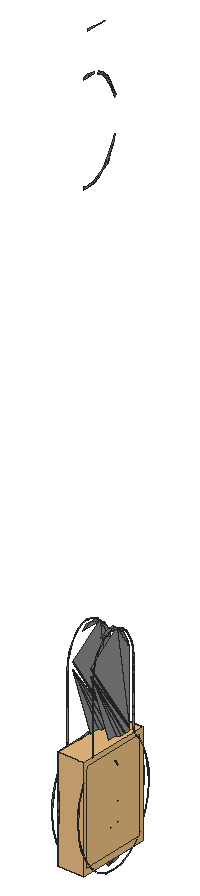
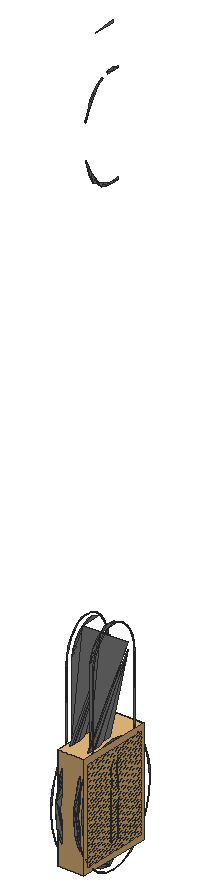
# SketchUp Ruby script. Lengths in inches.
U = 1.inch
M = Sketchup.active_model
def pt(a) = Geom::Point3d.new(a.map { |v| v * U })
def face(e, loops, mat)
  f = e.add_face(loops[0].map { |a| pt(a) })
  loops[1..].each { |l| e.add_face(l.map { |a| pt(a) }).erase! }
  f.material = f.back_material = mat if mat
  f
end
# faces: each face lists its corners as indices into pts; further lists are holes
def faces(e, pts, list, mat = nil) = list.each { |f| face(e, (f[0].is_a?(Array) ? f : [f]).map { |l| l.map { |i| pts[i] } }, mat) }
# xy, xz, yz: faces in a plane at the given z, y or x. An outline is a flat list of corners, or four numbers for a rectangle; further outlines are holes
def ring(l) = l.size == 4 ? [[l[0], l[1]], [l[2], l[1]], [l[2], l[3]], [l[0], l[3]]] : l.each_slice(2).to_a
def flat(e, list, mat, &to3) = list.each { |f| face(e, (f[0].is_a?(Array) ? f : [f]).map { |l| ring(l).map { |u, v| to3.(u, v) } }, mat) }
def xy(e, z, list, mat = nil) = flat(e, list, mat) { |x, y| [x, y, z] }
def xz(e, y, list, mat = nil) = flat(e, list, mat) { |x, z| [x, y, z] }
def yz(e, x, list, mat = nil) = flat(e, list, mat) { |y, z| [x, y, z] }
def lines(e, pts, list) = list.each { |a, b| e.add_line(pt(pts[a]), pt(pts[b])) }
# prism: a flat outline (further loops are holes) pulled along v
def prism(e, loops, v, mat = nil)
  f = face(e, loops, mat); d = Geom::Vector3d.new(v.map { |x| x * U })
  f.pushpull(f.normal.samedirection?(d) ? d.length : -d.length)
end
def box(e, o, s, mat = nil) = prism(e, [[o, [o[0] + s[0], o[1], o[2]], [o[0] + s[0], o[1] + s[1], o[2]], [o[0], o[1] + s[1], o[2]]]], [0, 0, s[2]], mat)
def at(x, y, z, deg = 0) = Geom::Transformation.translation(pt([x, y, z])) * Geom::Transformation.rotation(ORIGIN, Z_AXIS, deg.degrees)
def axes(o, x, y, z) = Geom::Transformation.new([*x, 0, *y, 0, *z, 0, *pt(o).to_a, 1])
def part(name) = M.definitions.add(name)
# library, detail: a bought-in or finely detailed component or shape, given as its bounding box
def library(name, o, s) = part(name).tap { |d| box(d.entities, o, s) }
def detail(e, o, s) = box(e.add_group.entities, o, s)
def put(e, d, t, mat = nil) = e.add_instance(d, t).tap { |i| i.material = mat if mat }
def group(e, t, mat = nil) = e.add_group.tap { |g| g.transformation = t; g.material = mat if mat }.entities
root = M.entities
M.materials.add("Material \#1").color = [140, 140, 140]
c1 = library("3DGeom~13_Defintion",[-84.91,-744.98,-830.03],[169.82,169.83,1000])
c2 = library("3DGeom~12_Defintion",[-95.68,-755.75,-830.03],[191.36,191.37,1000])
c3 = part("3DGeom~10_Defintion")
yz(c3.entities,-68.96,[[-797.08,-844.83,-797.08,-827.59,-922.41,-827.59],[-922.41,-844.83,-797.08,-844.83,-922.41,-827.59]],"Material \#1")
yz(c3.entities,68.97,[[-922.41,-844.83,-797.08,-827.59,-797.08,-844.83],[-922.41,-844.83,-922.41,-827.59,-797.08,-827.59],[-797.08,137.93,-922.41,155.17,-797.08,155.17],[-922.41,137.93,-922.41,155.17,-797.08,137.93]],"Material \#1")
p = [[-15.8,-989.55,-844.83],[-15.8,-989.55,-827.59],[0,-991.38,-827.59],[0,-991.38,-844.83],[15.8,-989.55,-827.59],[15.8,-989.55,-844.83],
  [-30.32,-984.36,-844.83],[-30.32,-984.36,-827.59],[30.31,-984.36,-827.59],[30.31,-984.36,-844.83],[-43.12,-976.21,-844.83],[-43.12,-976.21,-827.59],
  [43.12,-976.21,-827.59],[43.12,-976.21,-844.83],[-53.81,-965.53,-844.83],[-53.81,-965.53,-827.59],[53.8,-965.53,-827.59],[53.8,-965.53,-844.83],
  [-61.95,-952.73,-844.83],[-61.95,-952.73,-827.59],[53.8,-965.53,-827.59],[61.95,-952.73,-827.59],[61.95,-952.73,-844.83],[-67.15,-938.21,-844.83],
  [-67.15,-938.21,-827.59],[67.14,-938.21,-827.59],[67.14,-938.21,-844.83],[-68.96,-922.41,-844.83],[-68.96,-922.41,-827.59],[67.14,-938.21,-827.59],
  [68.97,-922.41,-827.59],[68.97,-922.41,-844.83],[-69.1,-794.86,-844.83],[-69.1,-794.86,-827.59],[-68.96,-797.08,-827.59],[-68.96,-797.08,-844.83],
  [68.97,-797.08,-844.83],[68.97,-797.08,-827.59],[69.11,-794.71,-827.59],[69.11,-794.71,-844.83],[-69.48,-792.73,-844.83],[-69.48,-792.73,-827.59],
  [69.53,-792.51,-827.59],[69.53,-792.51,-844.83],[-70.14,-790.6875,-844.83],[-70.14,-790.6875,-827.59],[70.24,-790.48,-827.59],[70.24,-790.48,-844.83],
  [-71.08,-788.73,-844.83],[-71.08,-788.73,-827.59],[71.22,-788.57,-827.59],[71.22,-788.57,-844.83],[-72.32,-786.86,-844.83],[-72.32,-786.86,-827.59],
  [72.47,-786.78,-827.59],[72.47,-786.78,-844.83],[-73.8,-785.17,-844.83],[-73.8,-785.17,-827.59],[74,-785.04,-827.59],[74,-785.04,-844.83],
  [-75.96,-783.21,-844.83],[-75.96,-783.21,-827.59],[74,-785.04,-827.59],[75.76,-783.39,-827.59],[75.76,-783.39,-844.83],[86.625,-772.95,-827.59],
  [86.61,-772.96,-844.83],[-86.89,-773.25,-844.83],[-86.89,-773.25,-827.59],[-75.96,-783.21,-844.83],[-96.66,-761.8,-844.83],[-96.66,-761.8,-827.59],
  [86.625,-772.95,-827.59],[86.63,-772.94,-844.83],[86.61,-772.96,-844.83],[86.625,-772.95,-827.59],[86.62,-772.95,-827.59],[86.62,-772.95,-827.59],
  [96.31,-761.375,-827.59],[96.31,-761.375,-844.83],[86.63,-772.94,-844.83],[86.625,-772.95,-827.59],[86.62,-772.95,-827.59],[-104.96,-749.18,-844.83],
  [-104.96,-749.18,-827.59],[-96.66,-761.8,-827.59],[-96.66,-761.8,-844.83],[96.31,-761.375,-827.59],[104.62,-748.77,-827.59],[104.62,-748.77,-844.83],
  [-111.64,-735.52,-844.83],[-111.64,-735.52,-827.59],[111.39,-735.21,-827.59],[111.39,-735.21,-844.83],[-116.49,-721.23,-844.83],[-116.49,-721.23,-827.59],
  [116.4375,-720.78,-827.59],[116.4375,-720.78,-844.83],[-119.64,-705.62,-844.83],[-119.64,-705.62,-827.59],[119.6,-705.57,-827.59],[119.6,-705.57,-844.83],
  [-120.6875,-689.65,-844.83],[-120.6875,-689.65,-827.59],[120.69,-689.65,-827.59],[120.69,-689.65,-844.83],[-117.5,-662,-844.83],[-117.5,-662,-827.59],
  [117.5,-662,-827.59],[117.5,-662,-844.83],[-108.41,-636.61,-844.83],[-108.41,-636.61,-827.59],[117.5,-662,-844.83],[108.41,-636.61,-827.59],
  [108.41,-636.61,-844.83],[-93.91,-613.95,-844.83],[-93.91,-613.95,-827.59],[-108.41,-636.61,-827.59],[108.41,-636.61,-844.83],[94.16,-614.19,-827.59],
  [94.16,-614.19,-844.83],[94.16,-614.19,-827.59],[75.46,-595.5,-827.59],[75.46,-595.5,-844.83],[-75.46,-595.5,-844.83],[-75.46,-595.5,-827.59],
  [-93.91,-613.95,-827.59],[-93.91,-613.95,-827.59],[-93.91,-613.95,-844.83],[-53.05,-581.24,-844.83],[-53.05,-581.24,-827.59],[-75.46,-595.5,-827.59],
  [-75.46,-595.5,-844.83],[53.05,-581.24,-827.59],[53.05,-581.24,-844.83],[-27.65,-572.16,-844.83],[-27.65,-572.16,-827.59],[-53.05,-581.24,-827.59],
  [-53.05,-581.24,-844.83],[27.66,-572.16,-827.59],[27.66,-572.16,-844.83],[0,-568.97,-844.83],[0,-568.97,-827.59],[-27.65,-572.16,-827.59],
  [-27.65,-572.16,-844.83],[0,-568.97,-844.83],[-15.8,-989.55,155.17],[0,-991.38,155.17],[0,-991.38,137.93],[-15.8,-989.55,137.93],
  [15.8,-989.55,155.17],[15.8,-989.55,137.93],[-30.32,-984.36,155.17],[-30.32,-984.36,137.93],[30.31,-984.36,155.17],[30.31,-984.36,137.93],
  [-43.125,-976.22,155.17],[-43.125,-976.22,137.93],[43.12,-976.22,155.17],[43.12,-976.22,137.93],[-53.81,-965.53,155.17],[-53.81,-965.53,137.93],
  [53.8,-965.53,155.17],[53.8,-965.53,137.93],[-61.96,-952.73,155.17],[-61.95,-952.73,137.93],[61.95,-952.73,155.17],[61.95,-952.73,137.93],
  [53.8,-965.53,137.93],[-67.15,-938.21,155.17],[-67.15,-938.21,137.93],[67.14,-938.21,155.17],[67.14,-938.21,137.93],[-68.96,-922.41,155.17],
  [-68.96,-922.41,137.93],[68.97,-922.41,155.17],[68.97,-922.41,137.93],[67.14,-938.21,137.93],[-68.97,-797.08,155.17],[-68.97,-797.08,137.93],
  [-69.1,-794.86,155.17],[-69.1,-794.86,137.93],[68.97,-797.08,155.17],[69.11,-794.71,155.17],[69.11,-794.71,137.93],[68.97,-797.08,137.93],
  [-69.48,-792.73,155.17],[-69.48,-792.73,137.93],[69.53,-792.51,155.17],[69.53,-792.51,137.93],[-70.14,-790.6875,155.17],[-70.14,-790.6875,137.93],
  [70.24,-790.48,155.17],[70.24,-790.48,137.93],[-71.08,-788.73,155.17],[-71.08,-788.73,137.93],[71.22,-788.57,155.17],[71.22,-788.57,137.93],
  [-72.32,-786.86,155.17],[-72.32,-786.86,137.93],[72.47,-786.78,155.17],[72.47,-786.78,137.93],[-73.8,-785.17,155.17],[-73.8,-785.17,137.93],
  [74,-785.04,155.17],[74,-785.04,137.93],[-75.96,-783.21,155.17],[-75.96,-783.21,137.93],[75.76,-783.39,155.17],[75.76,-783.39,137.93],
  [74,-785.04,137.93],[86.61,-772.96,155.17],[86.625,-772.95,137.93],[-86.88,-773.25,155.17],[-75.96,-783.21,155.17],[-86.88,-773.25,137.93],
  [-96.66,-761.8,155.17],[-96.66,-761.8,137.93],[86.63,-772.94,155.17],[86.625,-772.95,137.93],[86.61,-772.96,155.17],[86.62,-772.95,137.93],
  [86.625,-772.95,137.93],[96.31,-761.375,155.17],[96.31,-761.375,137.93],[86.62,-772.95,137.93],[86.63,-772.94,155.17],[86.62,-772.95,137.93],
  [86.625,-772.95,137.93],[-104.96,-749.18,155.17],[-96.66,-761.8,155.17],[-96.66,-761.8,137.93],[-104.96,-749.18,137.93],[104.62,-748.77,155.17],
  [104.62,-748.77,137.93],[96.31,-761.375,137.93],[-111.64,-735.52,155.17],[-111.64,-735.52,137.93],[111.39,-735.21,155.17],[111.39,-735.21,137.93],
  [-116.49,-721.23,155.17],[-116.49,-721.23,137.93],[116.4375,-720.78,155.17],[116.4375,-720.78,137.93],[-119.64,-705.62,155.17],[-119.64,-705.62,137.93],
  [119.6,-705.57,155.17],[119.6,-705.57,137.93],[-120.6875,-689.65,155.17],[-120.6875,-689.65,137.93],[120.69,-689.65,155.17],[120.69,-689.65,137.93],
  [-117.5,-662,155.17],[-117.5,-662,137.93],[117.5,-662,155.17],[117.5,-662,137.93],[-108.41,-636.61,155.17],[-108.41,-636.61,137.93],
  [117.5,-662,155.17],[108.41,-636.61,155.17],[108.41,-636.61,137.93],[-93.91,-613.95,155.17],[-108.41,-636.61,137.93],[-93.91,-613.95,137.93],
  [108.41,-636.61,155.17],[94.16,-614.19,155.17],[94.16,-614.19,137.93],[75.46,-595.5,155.17],[75.46,-595.5,137.93],[94.16,-614.19,137.93],
  [-75.46,-595.5,155.17],[-93.91,-613.95,155.17],[-93.91,-613.95,137.93],[-75.46,-595.5,137.93],[-53.05,-581.24,155.17],[-75.46,-595.5,155.17],
  [-75.46,-595.5,137.93],[-53.05,-581.24,137.93],[53.05,-581.24,155.17],[53.05,-581.24,137.93],[-27.65,-572.16,155.17],[-53.05,-581.24,155.17],
  [-53.05,-581.24,137.93],[-27.65,-572.16,137.93],[27.65,-572.16,155.17],[27.65,-572.16,137.93],[0,-568.97,155.17],[-27.65,-572.16,155.17],
  [-27.65,-572.16,137.93],[0,-568.97,137.93],[0,-568.97,155.17]]
faces(c3.entities,p,[[0,1,2],[2,3,0],[3,2,4],[4,5,3],[6,7,1],[1,0,6],[5,4,8],[8,9,5],
  [10,11,7],[7,6,10],[9,8,12],[12,13,9],[14,15,11],[11,10,14],[13,12,16],[16,17,13],
  [18,19,15],[15,14,18],[17,20,21],[21,22,17],[23,24,19],[19,18,23],[22,21,25],[25,26,22],
  [27,28,24],[24,23,27],[26,29,30],[30,31,26],[32,33,34],[34,35,32],[36,37,38],[38,39,36],
  [40,41,33],[33,32,40],[39,38,42],[42,43,39],[44,45,41],[41,40,44],[43,42,46],[46,47,43],
  [48,49,45],[45,44,48],[47,46,50],[50,51,47],[52,53,49],[49,48,52],[51,50,54],[54,55,51],
  [56,57,53],[53,52,56],[55,54,58],[58,59,55],[60,61,57],[57,56,60],[59,62,63],[63,64,59],
  [64,63,65],[65,66,64],[67,68,61],[61,69,67],[70,71,68],[68,67,70],[72,73,66],[74,75,76],
  [73,77,78],[78,79,73],[80,81,82],[83,84,85],[85,86,83],[79,87,88],[88,89,79],[90,91,84],
  [84,83,90],[89,88,92],[92,93,89],[94,95,91],[91,90,94],[93,92,96],[96,97,93],[98,99,95],
  [95,94,98],[97,96,100],[100,101,97],[102,103,99],[99,98,102],[101,100,104],[104,105,101],[106,107,103],
  [103,102,106],[105,104,108],[108,109,105],[110,111,107],[107,106,110],[112,108,113],[113,114,112],[115,116,117],
  [117,110,115],[118,113,119],[119,120,118],[120,121,122],[122,123,120],[124,125,126],[127,128,124],[129,130,131],
  [131,132,129],[123,122,133],[133,134,123],[135,136,137],[137,138,135],[134,133,139],[139,140,134],[141,142,143],
  [143,144,141],[140,139,142],[142,145,140],[146,147,148],[148,149,146],[147,150,151],[151,148,147],[152,146,149],
  [149,153,152],[150,154,155],[155,151,150],[156,152,153],[153,157,156],[154,158,159],[159,155,154],[160,156,157],
  [157,161,160],[158,162,163],[163,159,158],[164,160,161],[161,165,164],[162,166,167],[167,168,162],[169,164,165],
  [165,170,169],[166,171,172],[172,167,166],[173,169,170],[170,174,173],[171,175,176],[176,177,171],[178,173,174],
  [174,179,178],[180,178,179],[179,181,180],[182,183,184],[184,185,182],[186,180,181],[181,187,186],[183,188,189],
  [189,184,183],[190,186,187],[187,191,190],[188,192,193],[193,189,188],[194,190,191],[191,195,194],[192,196,197],
  [197,193,192],[198,194,195],[195,199,198],[196,200,201],[201,197,196],[202,198,199],[199,203,202],[200,204,205],
  [205,201,200],[206,202,203],[203,207,206],[204,208,209],[209,210,204],[208,211,212],[212,209,208],[213,214,207],
  [207,215,213],[216,213,215],[215,217,216],[211,218,219],[220,221,222],[218,223,224],[224,225,218],[226,227,228],
  [229,230,231],[231,232,229],[223,233,234],[234,235,223],[236,229,232],[232,237,236],[233,238,239],[239,234,233],
  [240,236,237],[237,241,240],[238,242,243],[243,239,238],[244,240,241],[241,245,244],[242,246,247],[247,243,242],
  [248,244,245],[245,249,248],[246,250,251],[251,247,246],[252,248,249],[249,253,252],[250,254,255],[255,251,250],
  [256,252,253],[253,257,256],[258,259,260],[260,255,258],[261,256,262],[262,263,261],[264,265,266],[266,260,264],
  [265,267,268],[268,269,265],[270,271,272],[272,273,270],[274,275,276],[276,277,274],[267,278,279],[279,268,267],
  [280,281,282],[282,283,280],[278,284,285],[285,279,278],[286,287,288],[288,289,286],[284,290,289],[289,285,284]],"Material \#1")
xy(root,57.581,[[155.634,443.997,155.634,444.049,155.657,444.049],[155.634,443.997,155.657,444.049,155.657,443.997]],"Material \#1")
xy(root,57.983,[[155.634,444.002,155.657,444.002,155.634,444.033],[155.657,444.002,155.657,444.033,155.634,444.033]],"Material \#1")
xz(root,443.994,[[155.634,57.78,155.657,57.78,155.634,57.809],[155.657,57.78,155.657,57.809,155.634,57.809]],"Material \#1")
xz(root,443.997,[[155.657,57.666,155.657,57.732,155.634,57.732]],"Material \#1")
xz(root,444.002,[[155.634,57.837,155.657,57.837,155.634,57.872],[155.657,57.837,155.657,57.872,155.634,57.872]],"Material \#1")
xz(root,444.044,[[155.634,57.872,155.657,57.91,155.657,57.872]],"Material \#1")
xz(root,444.049,[[155.634,57.581,155.657,57.646,155.657,57.581]],"Material \#1")
yz(root,155.637,[[444.023,60.855,444.023,60.87,443.986,60.86],[444.023,60.855,444.059,60.875,444.023,60.87],[444.023,60.855,444.061,60.86,444.059,60.875],[443.986,60.86,444.023,60.87,443.988,60.875],[444.061,60.86,444.092,60.888,444.059,60.875],
  [444.061,60.86,444.096,60.874,444.092,60.888],[444.096,60.874,444.123,60.908,444.092,60.888],[444.096,60.874,444.129,60.895,444.123,60.908],[444.129,60.895,444.151,60.936,444.123,60.908],[444.129,60.895,444.158,60.924,444.151,60.936],
  [444.158,60.924,444.175,60.969,444.151,60.936],[444.158,60.924,444.183,60.959,444.175,60.969],[444.183,60.959,444.195,61.008,444.175,60.969],[444.183,60.959,444.204,61,444.195,61.008],[444.204,61,444.209,61.051,444.195,61.008],
  [444.209,61.244,444.22,61.249,444.195,61.287],[444.22,61.249,444.204,61.295,444.195,61.287],[444.195,61.287,444.204,61.295,444.175,61.325],[444.204,61.295,444.183,61.335,444.175,61.325],[444.175,61.325,444.183,61.335,444.151,61.359],
  [444.183,61.335,444.158,61.37,444.151,61.359],[444.151,61.359,444.158,61.37,444.123,61.386],[444.158,61.37,444.129,61.399,444.123,61.386],[444.123,61.386,444.129,61.399,444.092,61.407],[444.129,61.399,444.096,61.421,444.092,61.407],
  [443.988,61.42,444.023,61.439,443.986,61.434],[443.988,61.42,444.023,61.424,444.023,61.439],[444.059,61.42,444.061,61.434,444.023,61.424],[444.023,61.424,444.061,61.434,444.023,61.439],[444.023,61.659,444.137,61.66,444.023,61.674]],"Material \#1")
yz(root,155.639,[[444.023,57.481,444.023,57.491,443.967,57.491],[444.023,57.481,444.077,57.501,444.023,57.491],[444.023,57.481,444.079,57.491,444.077,57.501],[443.967,57.491,443.969,57.501,443.915,57.521],[443.967,57.491,444.023,57.491,443.969,57.501],
  [444.079,57.491,444.128,57.53,444.077,57.501],[444.079,57.491,444.131,57.521,444.128,57.53],[443.969,57.501,443.919,57.53,443.915,57.521],[443.915,57.521,443.919,57.53,443.87,57.569],[444.131,57.521,444.171,57.576,444.128,57.53],
  [444.131,57.521,444.176,57.569,444.171,57.576],[443.919,57.53,443.875,57.576,443.87,57.569],[443.87,57.569,443.875,57.576,443.836,57.631],[444.176,57.569,444.204,57.636,444.171,57.576],[444.176,57.569,444.21,57.631,444.204,57.636],
  [443.875,57.576,443.842,57.636,443.836,57.631],[443.836,57.631,443.842,57.636,443.814,57.704],[444.21,57.631,444.225,57.707,444.204,57.636],[444.21,57.631,444.232,57.704,444.225,57.707],[443.842,57.636,443.821,57.707,443.814,57.704],
  [443.814,57.704,443.821,57.707,443.807,57.782],[444.232,57.704,444.232,57.782,444.225,57.707],[444.232,57.704,444.239,57.782,444.232,57.782],[443.821,57.707,443.814,57.782,443.807,57.782],[443.807,57.782,443.814,57.782,443.814,57.86],
  [443.814,57.782,443.821,57.857,443.814,57.86],[444.232,57.782,444.239,57.782,444.225,57.857],[444.239,57.782,444.232,57.86,444.225,57.857],[443.821,57.857,443.836,57.933,443.814,57.86],[443.821,57.857,443.842,57.928,443.836,57.933],
  [444.225,57.857,444.232,57.86,444.204,57.928],[444.232,57.86,444.21,57.933,444.204,57.928],[443.842,57.928,443.87,57.995,443.836,57.933],[443.842,57.928,443.875,57.988,443.87,57.995],[444.204,57.928,444.21,57.933,444.171,57.988],
  [444.21,57.933,444.176,57.995,444.171,57.988],[443.875,57.988,443.915,58.043,443.87,57.995],[443.875,57.988,443.919,58.034,443.915,58.043],[444.171,57.988,444.176,57.995,444.128,58.034],[444.176,57.995,444.131,58.043,444.128,58.034],
  [443.919,58.034,443.967,58.073,443.915,58.043],[443.919,58.034,443.969,58.063,443.967,58.073],[444.128,58.034,444.131,58.043,444.077,58.063],[444.131,58.043,444.079,58.073,444.077,58.063],[443.969,58.063,444.023,58.083,443.967,58.073],
  [443.969,58.063,444.023,58.073,444.023,58.083],[444.077,58.063,444.079,58.073,444.023,58.073],[444.023,58.073,444.079,58.073,444.023,58.083]],"Material \#1")
yz(root,155.657,[[443.997,57.581,444.049,57.581,444.049,57.646],[443.997,57.581,444.049,57.646,443.997,57.646],[443.997,57.646,444.043,57.651,444.003,57.651],[443.997,57.646,444.049,57.646,444.043,57.651],[444.003,57.651,444.043,57.651,444.043,57.661],
  [444.003,57.651,444.043,57.661,444.003,57.661],[444.003,57.661,444.049,57.666,443.997,57.666],[444.003,57.661,444.043,57.661,444.049,57.666],[443.997,57.666,444.049,57.666,444.049,57.732],[443.997,57.666,444.049,57.732,443.997,57.732],
  [443.997,57.732,444.044,57.752,444.002,57.752],[443.997,57.732,444.049,57.732,444.044,57.752],[444.002,57.752,444.052,57.78,443.994,57.78],[444.002,57.752,444.044,57.752,444.052,57.78],[443.994,57.78,444.052,57.78,444.052,57.809],
  [443.994,57.78,444.052,57.809,443.994,57.809],[443.994,57.809,444.044,57.837,444.002,57.837],[443.994,57.809,444.052,57.809,444.044,57.837],[444.002,57.837,444.044,57.837,444.044,57.872],[444.002,57.837,444.044,57.872,444.002,57.872],
  [444.002,57.872,444.044,57.872,444.044,57.91],[444.002,57.872,444.044,57.91,444.012,57.91],[444.012,57.91,444.049,57.92,444.007,57.92],[444.012,57.91,444.044,57.91,444.049,57.92],[444.007,57.92,444.049,57.92,444.049,57.943],
  [444.007,57.92,444.049,57.943,444.007,57.943],[444.007,57.943,444.044,57.953,444.012,57.953],[444.007,57.943,444.049,57.943,444.044,57.953],[444.012,57.953,444.033,57.983,444.002,57.983],[444.012,57.953,444.044,57.953,444.033,57.983]],"Material \#1")
yz(root,155.66,[[444.023,57.44,443.974,57.489,444.023,57.481],[444.023,57.44,444.023,57.481,444.073,57.489],[444.023,57.44,444.073,57.489,444.118,57.511],[444.023,57.44,444.118,57.511,444.214,57.568],[444.023,57.44,444.131,57.475,444.079,57.449],
  [444.023,57.44,444.214,57.568,444.131,57.475],[444.131,57.475,444.214,57.568,444.176,57.516],[444.118,57.511,444.158,57.547,444.214,57.568],[444.158,57.547,444.192,57.594,444.214,57.568],[444.214,57.568,444.192,57.594,444.217,57.65],
  [444.214,57.568,444.217,57.65,444.266,57.827],[444.214,57.568,444.262,57.704,444.243,57.632],[444.214,57.568,444.266,57.827,444.262,57.704],[444.217,57.65,444.234,57.713,444.266,57.827],[444.262,57.704,444.266,57.827,444.268,57.782],
  [444.234,57.713,444.239,57.782,444.266,57.827],[444.239,57.782,444.234,57.851,444.266,57.827],[444.266,57.827,444.165,58.066,444.168,58.059],[444.266,57.827,444.217,57.914,444.165,58.066],[444.266,57.827,444.168,58.059,444.172,58.053],
  [444.266,57.827,444.172,58.053,444.219,57.986],[444.266,57.827,444.234,57.851,444.217,57.914],[444.266,57.827,444.219,57.986,444.25,57.912],[444.266,57.827,444.25,57.912,444.26,57.871],[444.25,57.912,444.219,57.986,444.236,57.95],
  [444.217,57.914,444.192,57.97,444.165,58.066],[444.192,57.97,443.886,58.46,444.165,58.066],[444.192,57.97,444.158,58.017,443.886,58.46],[444.219,57.986,444.172,58.053,444.177,58.047],[444.219,57.986,444.177,58.047,444.2,58.019],
  [444.158,58.017,444.118,58.053,443.886,58.46],[444.118,58.053,444.073,58.075,443.886,58.46],[444.165,58.066,443.89,58.504,444.163,58.073],[444.163,58.073,443.89,58.504,444.161,58.08],[444.073,58.075,444.023,58.083,443.886,58.46],
  [444.161,58.08,443.89,58.504,444.16,58.087],[444.16,58.087,443.89,58.504,444.16,58.095],[444.16,58.095,443.89,58.504,444.083,58.631],[444.16,58.095,444.083,58.631,444.157,58.504],[444.16,58.095,444.157,58.504,444.16,58.46],
  [444.157,58.504,444.083,58.631,444.13,58.579],[444.157,58.504,444.13,58.579,444.146,58.544],[444.13,58.579,444.083,58.631,444.109,58.609],[444.083,58.631,443.963,58.632,444.023,58.651],[444.083,58.631,444.023,58.651,444.055,58.646],
  [443.963,58.632,443.992,58.646,444.023,58.651]],"Material \#1")
yz(root,155.76,[[444.023,57.44,444.023,57.481,443.974,57.489],[444.023,57.44,444.073,57.489,444.023,57.481],[444.023,57.44,444.079,57.449,444.131,57.475],[444.023,57.44,444.118,57.511,444.073,57.489],[444.023,57.44,444.131,57.475,444.214,57.568],
  [444.023,57.44,444.214,57.568,444.118,57.511],[444.131,57.475,444.176,57.516,444.214,57.568],[444.118,57.511,444.214,57.568,444.158,57.547],[444.158,57.547,444.214,57.568,444.192,57.594],[444.214,57.568,444.217,57.65,444.192,57.594],
  [444.214,57.568,444.243,57.632,444.262,57.704],[444.214,57.568,444.262,57.704,444.266,57.827],[444.214,57.568,444.266,57.827,444.217,57.65],[444.217,57.65,444.266,57.827,444.234,57.713],[444.262,57.704,444.268,57.782,444.266,57.827],
  [444.234,57.713,444.266,57.827,444.239,57.782],[444.239,57.782,444.266,57.827,444.234,57.851],[444.266,57.827,444.165,58.066,444.217,57.914],[444.266,57.827,444.168,58.059,444.165,58.066],[444.266,57.827,444.172,58.053,444.168,58.059],
  [444.266,57.827,444.219,57.986,444.172,58.053],[444.266,57.827,444.217,57.914,444.234,57.851],[444.266,57.827,444.25,57.912,444.219,57.986],[444.266,57.827,444.26,57.871,444.25,57.912],[444.25,57.912,444.236,57.95,444.219,57.986],
  [444.217,57.914,444.165,58.066,444.192,57.97],[444.192,57.97,443.886,58.46,444.158,58.017],[444.192,57.97,444.165,58.066,443.886,58.46],[444.219,57.986,444.177,58.047,444.172,58.053],[444.219,57.986,444.2,58.019,444.177,58.047],
  [444.158,58.017,443.886,58.46,444.118,58.053],[444.118,58.053,443.886,58.46,444.073,58.075],[444.165,58.066,444.163,58.073,443.89,58.504],[444.163,58.073,444.161,58.08,443.89,58.504],[444.073,58.075,443.886,58.46,444.023,58.083],
  [444.161,58.08,444.16,58.087,443.89,58.504],[444.16,58.087,444.16,58.095,443.89,58.504],[444.16,58.095,444.083,58.632,443.89,58.504],[444.16,58.095,444.157,58.504,444.083,58.632],[444.16,58.095,444.16,58.46,444.157,58.504],
  [444.157,58.504,444.13,58.579,444.083,58.632],[444.157,58.504,444.146,58.544,444.13,58.579],[444.13,58.579,444.109,58.609,444.083,58.632],[443.963,58.632,444.083,58.632,444.023,58.651],[444.083,58.632,444.055,58.646,444.023,58.651]],"Material \#1")
yz(root,155.763,[[443.997,57.581,443.997,57.646,444.049,57.646],[443.997,57.581,444.049,57.646,444.049,57.581],[443.997,57.646,444.003,57.651,444.043,57.651],[443.997,57.646,444.043,57.651,444.049,57.646],[444.003,57.651,444.003,57.661,444.043,57.661],
  [444.003,57.651,444.043,57.661,444.043,57.651],[444.003,57.661,443.997,57.666,444.049,57.666],[444.003,57.661,444.049,57.666,444.043,57.661],[443.997,57.666,443.997,57.732,444.049,57.732],[443.997,57.666,444.049,57.732,444.049,57.666],
  [443.997,57.732,444.002,57.752,444.044,57.752],[443.997,57.732,444.044,57.752,444.049,57.732],[444.002,57.752,443.994,57.78,444.052,57.78],[444.002,57.752,444.052,57.78,444.044,57.752],[443.994,57.78,443.994,57.809,444.052,57.809],
  [443.994,57.78,444.052,57.809,444.052,57.78],[443.994,57.809,444.002,57.837,444.044,57.837],[443.994,57.809,444.044,57.837,444.052,57.809],[444.002,57.837,444.002,57.872,444.044,57.872],[444.002,57.837,444.044,57.872,444.044,57.837],
  [444.002,57.872,444.012,57.91,444.044,57.91],[444.002,57.872,444.044,57.91,444.044,57.872],[444.012,57.91,444.007,57.92,444.049,57.92],[444.012,57.91,444.049,57.92,444.044,57.91],[444.007,57.92,444.007,57.943,444.049,57.943],
  [444.007,57.92,444.049,57.943,444.049,57.92],[444.007,57.943,444.012,57.953,444.044,57.953],[444.007,57.943,444.044,57.953,444.049,57.943],[444.012,57.953,444.002,57.983,444.033,57.983],[444.012,57.953,444.033,57.983,444.044,57.953]],"Material \#1")
p = [[155.634,444.049,57.581],[155.634,444.047,57.661],[155.657,444.049,57.646],[155.634,444,57.654],[155.634,443.997,57.581],[155.657,443.997,57.581],
  [155.657,443.997,57.581],[155.657,443.997,57.646],[155.634,444,57.654],[155.634,444.047,57.661],[155.657,444.043,57.651],[155.657,444.049,57.646],
  [155.634,444,57.654],[155.657,443.997,57.646],[155.657,444.003,57.651],[155.786,444.047,57.661],[155.763,444.049,57.646],[155.763,444.043,57.651],
  [155.786,444,57.654],[155.763,444.003,57.651],[155.763,443.997,57.646],[155.634,444.046,57.742],[155.634,444.048,57.766],[155.657,444.052,57.78],
  [155.634,444.049,57.727],[155.634,444.046,57.742],[155.657,444.044,57.752],[155.634,444.047,57.661],[155.634,444.049,57.727],[155.657,444.049,57.732],
  [155.634,443.997,57.732],[155.634,444,57.654],[155.657,443.997,57.666],[155.634,444.002,57.752],[155.634,443.997,57.732],[155.657,443.997,57.732],
  [155.657,444.052,57.78],[155.657,444.044,57.752],[155.634,444.046,57.742],[155.657,444.044,57.752],[155.657,444.049,57.732],[155.634,444.049,57.727],
  [155.657,444.049,57.732],[155.657,444.049,57.666],[155.634,444.047,57.661],[155.657,443.997,57.732],[155.657,444.002,57.752],[155.634,444.002,57.752],
  [155.634,444,57.654],[155.657,444.003,57.661],[155.657,443.997,57.666],[155.634,444.047,57.661],[155.657,444.043,57.661],[155.634,444.047,57.661],
  [155.657,444.049,57.666],[155.634,444,57.654],[155.786,444,57.654],[155.763,443.997,57.666],[155.763,444.003,57.661],[155.786,444.047,57.661],
  [155.763,444.043,57.661],[155.786,444.047,57.661],[155.763,444.049,57.666],[155.786,444,57.654],[155.634,444.048,57.823],[155.634,444.044,57.872],
  [155.657,444.044,57.872],[155.634,444.052,57.795],[155.634,444.048,57.823],[155.657,444.044,57.837],[155.634,444.048,57.766],[155.634,444.052,57.795],
  [155.657,444.052,57.809],[155.634,443.994,57.78],[155.634,444.002,57.752],[155.657,444.002,57.752],[155.634,444.002,57.837],[155.634,443.994,57.809],
  [155.657,443.994,57.809],[155.657,444.002,57.837],[155.657,444.044,57.872],[155.657,444.044,57.837],[155.634,444.048,57.823],[155.657,444.044,57.837],
  [155.657,444.052,57.809],[155.634,444.052,57.795],[155.657,444.052,57.809],[155.657,444.052,57.78],[155.634,444.048,57.766],[155.657,444.002,57.752],
  [155.657,443.994,57.78],[155.634,443.994,57.78],[155.786,444.048,57.766],[155.763,444.052,57.78],[155.763,444.052,57.809],[155.634,444.044,57.872],
  [155.634,444.046,57.915],[155.657,444.044,57.91],[155.634,444.002,57.983],[155.634,444.01,57.948],[155.657,444.012,57.953],[155.634,444.01,57.915],
  [155.634,444.002,57.872],[155.657,444.002,57.872],[155.634,444.046,57.915],[155.634,444.046,57.948],[155.657,444.049,57.943],[155.657,444.049,57.92],
  [155.634,444.01,57.948],[155.634,444.01,57.915],[155.657,444.007,57.92],[155.657,444.007,57.943],[155.634,444.046,57.948],[155.657,444.044,57.953],
  [155.657,444.049,57.943],[155.634,444.046,57.915],[155.657,444.049,57.92],[155.657,444.044,57.91],[155.634,444.01,57.948],[155.657,444.007,57.943],
  [155.657,444.012,57.953],[155.634,444.01,57.915],[155.657,444.012,57.91],[155.657,444.007,57.92],[155.657,444.002,57.872],[155.657,444.012,57.91],
  [155.634,444.01,57.915],[155.634,444.046,57.948],[155.634,444.033,57.983],[155.657,444.033,57.983],[155.657,444.044,57.953],[155.634,444.046,57.948],
  [155.786,444.046,57.948],[155.763,444.044,57.953],[155.763,444.033,57.983],[155.786,444.033,57.983],[155.786,444.046,57.948],[155.657,444.012,57.953],
  [155.657,444.002,57.983],[155.634,444.002,57.983],[155.637,443.951,61.0625],[155.637,443.935,61.031],[155.639,443.935,61.031],[155.639,443.951,61.0625],
  [155.637,443.953,61.008],[155.639,443.953,61.008],[155.637,443.975,60.992],[155.639,443.975,60.992],[155.637,443.991,61.024],[155.639,443.991,61.024],
  [155.637,444.005,61.052],[155.639,444.005,61.052],[155.637,443.965,61.091],[155.639,443.965,61.091],[155.637,444.081,61.204],[155.639,444.081,61.204],
  [155.637,444.041,61.243],[155.639,444.041,61.243],[155.637,444.055,61.271],[155.639,444.055,61.271],[155.637,444.095,61.232],[155.639,444.095,61.232],
  [155.637,444.111,61.263],[155.639,444.111,61.263],[155.637,444.093,61.286],[155.639,444.093,61.286],[155.637,444.071,61.302],[155.639,444.071,61.302]]
faces(root,p,[[0,1,2],[3,4,5],[6,7,8],[9,10,11],[12,13,14],[15,16,17],[18,19,20],[21,22,23],
  [24,25,26],[27,28,29],[30,31,32],[33,34,35],[36,37,38],[39,40,41],[42,43,44],[45,46,47],
  [48,49,50],[51,52,10],[53,54,52],[55,14,49],[56,57,58],[59,17,60],[61,60,62],[63,58,19],
  [64,65,66],[67,68,69],[70,71,72],[73,74,75],[76,77,78],[78,79,76],[80,81,82],[83,84,85],
  [86,87,88],[89,90,91],[92,93,94],[95,96,97],[98,99,100],[101,102,103],[104,105,106],[106,107,104],
  [108,109,110],[110,111,108],[112,113,114],[115,116,117],[118,119,120],[121,122,123],[124,125,126],[127,128,129],
  [129,130,131],[132,133,134],[134,135,136],[137,138,139],[140,141,142],[142,143,140],[141,144,145],[145,142,141],
  [144,146,147],[147,145,144],[146,148,149],[149,147,146],[148,150,151],[151,149,148],[152,140,143],[143,153,152],
  [150,154,155],[155,151,150],[156,152,153],[153,157,156],[158,156,157],[157,159,158],[154,160,161],[161,155,154],
  [160,162,163],[163,161,160],[162,164,165],[165,163,162],[164,166,167],[167,165,164],[166,158,159],[159,167,166]],"Material \#1")
put(root,c1,axes([155.66,444.02,55.77],[0,-0.00218,0],[0,0,-0.00304],[-0.00015,0,0]),"Material \#1")
put(root,c2,axes([155.66,444.02,55.77],[0,-0.00218,0],[0,0,-0.00304],[-0.00015,0,0]),"Material \#1")
put(root,c3,axes([155.66,444.02,55.77],[0,-0.00209,0],[0,0,-0.00291],[-0.00015,0,0]),"Material \#1")
